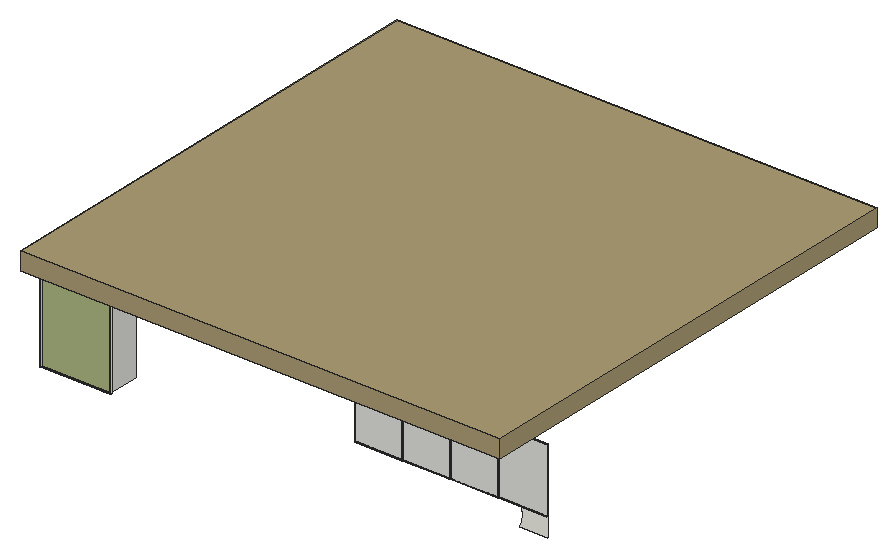
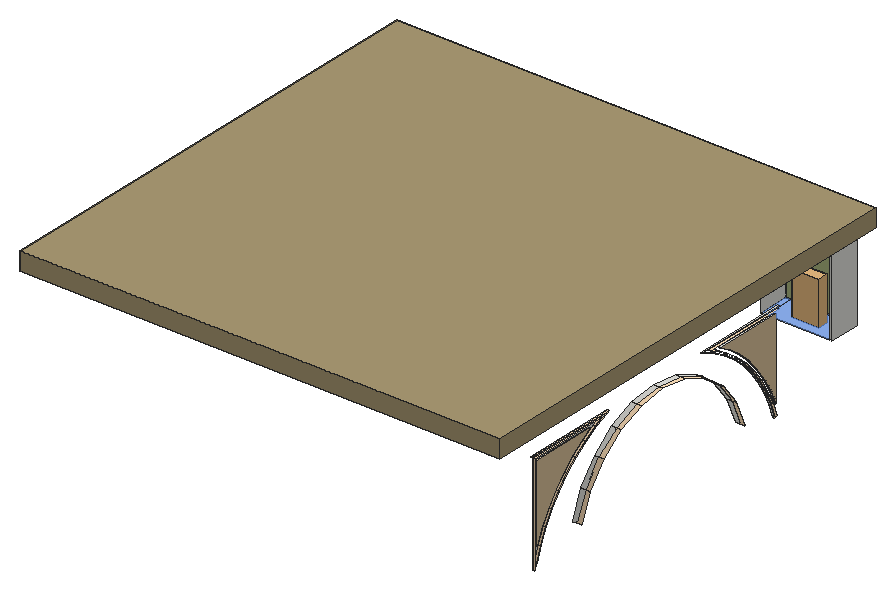
# SketchUp Ruby script. Lengths in inches.
U = 1.inch
M = Sketchup.active_model
def pt(a) = Geom::Point3d.new(a.map { |v| v * U })
def face(e, loops, mat)
  f = e.add_face(loops[0].map { |a| pt(a) })
  loops[1..].each { |l| e.add_face(l.map { |a| pt(a) }).erase! }
  f.material = f.back_material = mat if mat
  f
end
# faces: each face lists its corners as indices into pts; further lists are holes
def faces(e, pts, list, mat = nil) = list.each { |f| face(e, (f[0].is_a?(Array) ? f : [f]).map { |l| l.map { |i| pts[i] } }, mat) }
# xy, xz, yz: faces in a plane at the given z, y or x. An outline is a flat list of corners, or four numbers for a rectangle; further outlines are holes
def ring(l) = l.size == 4 ? [[l[0], l[1]], [l[2], l[1]], [l[2], l[3]], [l[0], l[3]]] : l.each_slice(2).to_a
def flat(e, list, mat, &to3) = list.each { |f| face(e, (f[0].is_a?(Array) ? f : [f]).map { |l| ring(l).map { |u, v| to3.(u, v) } }, mat) }
def xy(e, z, list, mat = nil) = flat(e, list, mat) { |x, y| [x, y, z] }
def xz(e, y, list, mat = nil) = flat(e, list, mat) { |x, z| [x, y, z] }
def yz(e, x, list, mat = nil) = flat(e, list, mat) { |y, z| [x, y, z] }
def lines(e, pts, list) = list.each { |a, b| e.add_line(pt(pts[a]), pt(pts[b])) }
# prism: a flat outline (further loops are holes) pulled along v
def prism(e, loops, v, mat = nil)
  f = face(e, loops, mat); d = Geom::Vector3d.new(v.map { |x| x * U })
  f.pushpull(f.normal.samedirection?(d) ? d.length : -d.length)
end
def box(e, o, s, mat = nil) = prism(e, [[o, [o[0] + s[0], o[1], o[2]], [o[0] + s[0], o[1] + s[1], o[2]], [o[0], o[1] + s[1], o[2]]]], [0, 0, s[2]], mat)
def at(x, y, z, deg = 0) = Geom::Transformation.translation(pt([x, y, z])) * Geom::Transformation.rotation(ORIGIN, Z_AXIS, deg.degrees)
def axes(o, x, y, z) = Geom::Transformation.new([*x, 0, *y, 0, *z, 0, *pt(o).to_a, 1])
def part(name) = M.definitions.add(name)
# library, detail: a bought-in or finely detailed component or shape, given as its bounding box
def library(name, o, s) = part(name).tap { |d| box(d.entities, o, s) }
def detail(e, o, s) = box(e.add_group.entities, o, s)
def put(e, d, t, mat = nil) = e.add_instance(d, t).tap { |i| i.material = mat if mat }
def group(e, t, mat = nil) = e.add_group.tap { |g| g.transformation = t; g.material = mat if mat }.entities
root = M.entities
M.materials.add("BACK Wall colour").color = [219, 194, 155]
M.materials.add("Emissive").color = [255, 225, 187]
M.materials.add("Emissive\#1").color = [255, 255, 255]
M.materials.add("[Color A01]").color = [173, 157, 118]
M.materials.add("[Translucent Glass Blue]").color = [100, 149, 237]
M.materials["[Translucent Glass Blue]"].alpha = 0.5
M.materials.add("celling colour").color = [232, 202, 161]
M.materials.add("cubod").color = [174, 185, 130]
M.materials.add("cubod wall").color = [240, 240, 232]
c1 = library("Group\#137",[0,0,0],[10.08,3.9375,16.2])
c2 = library("Ceiling Lamp 298 005",[-48.92,-48.77,-111.12],[97.53,97.41,111.46])
c3 = part("Component\#3")
detail(c3.entities,[-0.59,-0.59,-1.4375],[11.52,11.52,1.6875])
xy(root,93.69,[[688.79,27,706.63,27.75],[706.79,27,724.63,27.75]])
xy(root,94,[[589.4375,4,613.52,4.375],[613.52,4,615.39,4.375],[688.79,27,706.63,27.75],[706.79,27,724.63,27.75],[724.63,27,724.79,27.75]])
xy(root,94,[[589.4375,4.375,613.52,16],[613.52,4.375,615.39,16]],"[Translucent Glass Blue]")
xy(root,94.39,[[589.4375,4,615.39,4.375]])
xy(root,94.39,[[589.4375,4.375,615.39,16]],"[Translucent Glass Blue]")
xy(root,115.1875,[[588.45,43.01,588.79,68.75],[588.42,130.16,588.79,155.1875]])
xy(root,115.1875,[[588.1,43.01,588.45,68.75],[588.1,130.16,588.42,155.1875]],"Emissive")
xy(root,116.375,[[588.1,41.82,588.79,73.63],[588.1,125.18,588.79,156.375]],"Emissive")
xy(root,117.17,[[588.45,41.03,588.79,77.31],[588.45,121.42,588.79,157.17]])
xy(root,117.17,[[588.1,41.03,588.45,77.31],[588.1,121.42,588.45,157.17]],"Emissive")
xy(root,118,[[688.79,27,706.63,27.75],[706.79,27,724.63,27.75],[724.79,27,742.63,27.75],[742.79,27,760.79,27.75]])
xy(root,124,[[588.79,4,589.4375,16],[589.4375,4,615.39,4.375],[615.39,4,616.04,4.375],[615.39,4.375,616.04,16]])
xy(root,124,[[589.4375,4.375,615.39,16]],"[Translucent Glass Blue]")
xy(root,124.2,[[588.79,4,589.4375,4.375],[589.4375,4,616.04,4.375]])
xy(root,124.57,[[589.4375,4,616.04,16]],"[Translucent Glass Blue]")
xy(root,126.48,[[584.79,4,588.79,176.875]])
xz(root,4,[[589.4375,94,615.39,94.39],[615.39,94.39,616.04,124],[588.79,124,589.4375,124.2],[589.4375,124,616.04,124.2],[589.4375,124.2,616.04,124.57]])
xz(root,4.375,[[589.4375,94.39,615.39,124]],"cubod")
xz(root,16,[[589.4375,124,616.04,124.57]],"[Translucent Glass Blue]")
xz(root,27,[[688.79,93.69,706.79,94],[706.79,93.69,724.79,94],[724.79,93.69,742.63,94],[742.63,93.69,742.79,94],[742.79,93.69,760.79,94],
  [688.79,94,706.63,118],[706.63,94,706.79,118],[706.79,94,724.63,118],[724.63,94,724.79,118],[724.79,94,742.63,118],
  [742.63,94,742.79,118],[742.79,94,760.79,118]])
xz(root,27.75,[[688.79,94,688.79,100.05,688.86,100.89,689.08,101.7,689.44,102.46,689.93,103.15,690.53,103.74,691.23,104.22,691.99,104.56,692.81,104.77,693.65,104.83,694.49,104.75,695.3,104.51,696.05,104.14,696.4,106.79,697.42,109.25,699.04,111.37,701.16,112.99,703.625,114.01,706.27,114.36,706.63,114.32,706.63,94],[706.79,94,706.79,114.29,708.92,114.01,711.38,112.99,713.5,111.37,715.12,109.25,716.14,106.79,716.49,104.14,717.99,106.42,720.03,108.23,722.47,109.44,724.63,109.89,724.63,94]],"cubod")
xz(root,27.75,[[750.1,86.35,750.97,88.41,751.28,90.64,750.99,92.86,750.15,94.9375,748.79,96.73,747.02,98.1,744.95,98.97,742.79,99.26,742.79,118,760.79,118,760.79,86.35],[735.26,95.01,736.125,97.6,736.29,100.32,735.74,102.99,734.52,105.42,732.71,107.46,730.44,108.97,727.86,109.83,725.14,109.99,724.79,109.92,724.79,118,742.63,118,742.63,99.26,740.5,98.99,738.42,98.14,736.64,96.79],[688.79,100.05,688.79,118,706.63,118,706.63,114.32,706.27,114.36,703.625,114.01,701.16,112.99,699.04,111.37,697.42,109.25,696.4,106.79,696.05,104.14,695.3,104.51,694.49,104.75,693.65,104.83,692.81,104.77,691.99,104.56,691.23,104.22,690.53,103.74,689.93,103.15,689.44,102.46,689.08,101.7,688.86,100.89],[716.49,104.14,716.14,106.79,715.12,109.25,713.5,111.37,711.38,112.99,708.92,114.01,706.79,114.29,706.79,118,724.63,118,724.63,109.89,722.47,109.44,720.03,108.23,717.99,106.42]],"cubod wall")
xz(root,43.01,[[588.45,85.13,588.79,115.1875]])
xz(root,43.01,[[588.1,85.13,588.45,115.1875]],"Emissive")
xz(root,155.1875,[[588.42,86.57,588.79,115.1875]])
xz(root,155.1875,[[588.1,86.57,588.42,115.1875]],"Emissive")
xz(root,156.375,[[588.1,78.67,588.79,116.375]],"Emissive")
yz(root,588.1,[[43.01,85.13,43.52,86.57,45.99,91.8,48.96,96.77,52.41,101.42,56.29,105.71,60.57,109.6,65.21,113.06,68.75,115.1875,43.01,115.1875],[155.1875,86.57,155.1875,115.1875,130.16,115.1875,133.5625,113.1875,138.23,109.76,142.53,105.87,146.41,101.57,149.84,96.89,152.77,91.89,155.17,86.62]],"BACK Wall colour")
yz(root,588.79,[[[156.375,78.67,156.375,116.375,125.18,116.375,128.02,115.07,132.91,112.2,137.48,108.84,141.69,105.03,145.49,100.82,148.84,96.24,151.71,91.34,154.07,86.18,155.89,80.81],[155.1875,86.57,155.17,86.62,152.77,91.89,149.84,96.89,146.41,101.57,142.53,105.87,138.23,109.76,133.5625,113.1875,130.16,115.1875,155.1875,115.1875]],[4,94,16,124],[4,124,16,124.2],[4,124.2,16,126.48]])
yz(root,589.4375,[[4,94.39,4.375,124],[4.375,94.39,16,124],[4.375,124,4.375,124.2,4,124.2,4,124.57,16,124.57,16,124]])
yz(root,615.39,[[4,94.39,4.375,124],[4.375,94.39,16,124]])
yz(root,616.04,[[4,124,16,124.2],[4,124.2,16,124.57]],"[Translucent Glass Blue]")
yz(root,688.79,[[27,94,27.75,118]])
yz(root,706.63,[[27,94,27.75,118]])
yz(root,706.79,[[27,94,27.75,118]])
yz(root,724.63,[[27,94,27.75,118]])
yz(root,724.79,[[27,93.69,27.75,94],[27,94,27.75,118]])
yz(root,742.63,[[27,93.69,27.75,94],[27,94,27.75,118]])
yz(root,742.79,[[27,93.69,27.75,94],[27,94,27.75,118]])
p = [[588.79,156.375,78.67],[588.79,155.89,80.81],[588.1,155.89,80.81],[588.1,156.375,78.67],[588.1,43.48,80.54],[588.45,43.48,80.54],
  [588.45,45.36,85.81],[588.1,45.36,85.81],[588.79,45.36,85.81],[588.79,43.48,80.54],[588.1,153.33,85.89],[588.45,153.33,85.89],
  [588.45,155.12,80.59],[588.1,155.12,80.59],[588.79,155.12,80.59],[588.79,153.33,85.89],[588.79,44.62,86.11],[588.79,42.71,80.77],
  [588.1,42.71,80.77],[588.1,44.62,86.11],[588.79,154.07,86.18],[588.1,154.07,86.18],[588.1,43.01,85.13],[588.45,43.01,85.13],
  [588.45,43.52,86.57],[588.1,43.52,86.57],[588.79,43.52,86.57],[588.79,43.01,85.13],[588.45,47.74,90.87],[588.1,47.74,90.87],
  [588.79,47.74,90.87],[588.1,151,90.98],[588.45,151,90.98],[588.79,151,90.98],[588.79,47.04,91.24],[588.1,47.04,91.24],
  [588.79,151.71,91.34],[588.1,151.71,91.34],[588.45,45.99,91.8],[588.1,45.99,91.8],[588.79,45.99,91.8],[588.1,152.77,91.89],
  [588.42,152.77,91.89],[588.42,155.17,86.62],[588.1,155.17,86.62],[588.79,155.17,86.62],[588.79,152.77,91.89],[588.42,155.1875,86.57],
  [588.1,155.1875,86.57],[588.79,155.1875,86.57],[585.35,65.14,96.27],[587.07,65.14,96.27],[587.07,61.19,86.73],[585.35,61.19,86.73],
  [588.79,61.19,86.73],[588.79,65.14,96.27],[585.35,137.54,86.73],[587.07,137.54,86.73],[587.07,133.59,96.27],[585.35,133.59,96.27],
  [588.79,133.59,96.27],[588.79,137.54,86.73],[588.45,50.61,95.67],[588.1,50.61,95.67],[588.79,50.61,95.67],[588.1,148.18,95.8],
  [588.45,148.18,95.8],[588.79,148.18,95.8],[588.79,49.95,96.11],[588.1,49.95,96.11],[588.79,148.84,96.24],[588.1,148.84,96.24],
  [588.45,48.96,96.77],[588.1,48.96,96.77],[588.79,48.96,96.77],[588.1,149.84,96.89],[588.42,149.84,96.89],[588.79,149.84,96.89],
  [588.45,53.94,100.16],[588.1,53.94,100.16],[588.79,53.94,100.16],[588.1,144.87,100.31],[588.45,144.87,100.31],[588.79,144.87,100.31],
  [588.79,53.33,100.67],[588.1,53.33,100.67],[588.79,145.49,100.82],[588.1,145.49,100.82],[585.35,71.42,104.45],[587.07,71.42,104.45],
  [588.79,71.42,104.45],[587.07,127.31,104.45],[585.35,127.31,104.45],[588.79,127.31,104.45],[588.45,52.41,101.42],[588.1,52.41,101.42],
  [588.79,52.41,101.42],[588.1,146.41,101.57],[588.42,146.41,101.57],[588.79,146.41,101.57],[588.45,57.69,104.3125],[588.1,57.69,104.3125],
  [588.79,57.69,104.3125],[588.1,141.13,104.47],[588.45,141.13,104.47],[588.79,141.13,104.47],[588.79,57.13,104.875],[588.1,57.13,104.875],
  [588.79,141.69,105.03],[588.1,141.69,105.03],[588.45,56.29,105.71],[588.1,56.29,105.71],[588.79,56.29,105.71],[588.1,142.53,105.87],
  [588.42,142.53,105.87],[588.79,142.53,105.87],[588.45,61.83,108.07],[588.1,61.83,108.07],[588.79,61.83,108.07],[585.35,79.6,110.73],
  [587.07,79.6,110.73],[588.79,79.6,110.73],[587.07,119.125,110.73],[585.35,119.125,110.73],[588.79,119.125,110.73],[588.1,136.98,108.22],
  [588.45,136.98,108.22],[588.79,136.98,108.22],[588.79,61.32,108.6875],[588.1,61.32,108.6875],[588.79,137.48,108.84],[588.1,137.48,108.84],
  [588.45,60.57,109.6],[588.1,60.57,109.6],[588.79,60.57,109.6],[588.1,138.23,109.76],[588.42,138.23,109.76],[588.79,138.23,109.76],
  [588.45,66.32,111.41],[588.1,66.32,111.41],[588.79,66.32,111.41],[588.1,132.47,111.53],[588.45,132.47,111.53],[588.79,132.47,111.53],
  [588.79,65.875,112.07],[588.1,65.875,112.07],[588.79,132.91,112.2],[588.1,132.91,112.2],[588.45,65.21,113.06],[588.1,65.21,113.06],
  [588.79,65.21,113.06],[588.1,133.5625,113.1875],[588.42,133.5625,113.1875],[588.79,133.5625,113.1875],[585.35,89.14,114.68],[587.07,89.14,114.68],
  [588.79,89.14,114.68],[587.07,109.59,114.68],[585.35,109.59,114.68],[588.79,109.59,114.68],[588.45,71.11,114.29],[588.1,71.11,114.29],
  [588.79,71.11,114.29],[588.1,127.65,114.37],[588.45,127.65,114.37],[588.79,127.65,114.37],[588.79,70.73,115],[588.1,70.73,115],
  [588.79,128.02,115.07],[588.1,128.02,115.07],[588.45,68.75,115.1875],[588.1,68.75,115.1875],[588.79,68.75,115.1875],[588.1,130.16,115.1875],
  [588.42,130.16,115.1875],[588.79,130.16,115.1875],[588.45,76.16,116.7],[588.1,76.16,116.7],[588.79,76.16,116.7],[588.1,122.57,116.7],
  [588.45,122.57,116.7],[588.79,122.57,116.7],[585.35,99.36,116.03],[587.07,99.36,116.03],[588.79,99.36,116.03],[588.79,73.63,116.375],
  [588.1,73.63,116.375],[588.79,125.18,116.375],[588.1,125.18,116.375],[588.45,77.31,117.17],[588.1,77.31,117.17],[588.79,77.31,117.17],
  [588.1,121.42,117.17],[588.45,121.42,117.17],[588.79,121.42,117.17],[724.79,27.75,109.92],[724.63,27.75,109.89],[706.79,27.75,114.29],
  [706.63,27.75,114.32],[742.73,27.75,99.27],[742.63,27.75,99.26],[742.79,27.75,99.26],[742.63,27.75,118],[742.79,27.75,118]]
faces(root,p,[[0,1,2,3],[4,5,6,7],[10,11,12,13],[16,17,18,19],[1,20,21,2],[22,23,24,25],[7,6,28,29],[31,32,11,10],
  [34,16,19,35],[20,36,37,21],[25,24,38,39],[41,42,43,44],[44,43,47,48],[50,51,52,53],[56,57,58,59],[29,28,62,63],
  [65,66,32,31],[68,34,35,69],[36,70,71,37],[39,38,72,73],[75,76,42,41],[63,62,78,79],[81,82,66,65],[84,68,69,85],
  [70,86,87,71],[88,89,51,50],[59,58,91,92],[73,72,94,95],[97,98,76,75],[79,78,100,101],[103,104,82,81],[106,84,85,107],
  [86,108,109,87],[95,94,110,111],[113,114,98,97],[101,100,116,117],[119,120,89,88],[92,91,122,123],[125,126,104,103],[128,106,107,129],
  [108,130,131,109],[111,110,132,133],[135,136,114,113],[117,116,138,139],[141,142,126,125],[144,128,129,145],[130,146,147,131],[133,132,148,149],
  [151,152,136,135],[154,155,120,119],[123,122,157,158],[139,138,160,161],[163,164,142,141],[166,144,145,167],[146,168,169,147],[149,148,170,171],
  [173,174,152,151],[161,160,176,177],[179,180,164,163],[182,183,155,154],[158,157,183,182],[185,166,167,186],[168,187,188,169],[177,176,189,190],
  [192,193,180,179]],"Emissive")
faces(root,p,[[8,6,5,9],[14,12,11,15],[26,24,23,27],[30,28,6,8],[15,11,32,33],[40,38,24,26],[45,43,42,46],[49,47,43,45],
  [54,52,51,55],[60,58,57,61],[64,62,28,30],[33,32,66,67],[74,72,38,40],[46,42,76,77],[80,78,62,64],[67,66,82,83],
  [55,51,89,90],[93,91,58,60],[96,94,72,74],[77,76,98,99],[102,100,78,80],[83,82,104,105],[112,110,94,96],[99,98,114,115],
  [118,116,100,102],[90,89,120,121],[124,122,91,93],[105,104,126,127],[134,132,110,112],[115,114,136,137],[140,138,116,118],[127,126,142,143],
  [150,148,132,134],[137,136,152,153],[121,120,155,156],[159,157,122,124],[162,160,138,140],[143,142,164,165],[172,170,148,150],[153,152,174,175],
  [178,176,160,162],[165,164,180,181],[156,155,183,184],[184,183,157,159],[191,189,176,178],[181,180,193,194]])
lines(root,p,[[195,196],[197,198],[199,200],[201,199],[202,203]])
put(root,c1,at(606.5,12.53,94.39,180))
put(root,c2,axes([663.66,98.67,131.84],[0.279,0,0],[0,0.279,0],[0,0,0.279]))
g1 = group(root,at(588.79,23.29,135.52),"[Color A01]")
xy(g1,-9.04,[[[-4,-23.29,176,153.59],[24.9375,23.99,24.49,24.02,24.04,24.1,23.62,24.25,23.21,24.45,22.84,24.7,22.5,25,22.2,25.34,21.95,25.71,21.75,26.12,21.6,26.55,21.51,26.99,21.48,27.44,21.48,127.94,21.51,128.39,21.6,128.84,21.75,129.26,21.95,129.67,22.2,130.04,22.5,130.38,22.84,130.68,23.21,130.93,23.62,131.13,24.04,131.28,24.49,131.37,24.9375,131.4,136.36,131.4,136.81,131.37,137.25,131.28,137.68,131.13,138.09,130.93,138.46,130.68,138.8,130.38,139.1,130.04,139.35,129.67,139.55,129.26,139.7,128.84,139.78,128.39,139.8125,127.94,139.8125,27.44,139.78,26.99,139.7,26.55,139.55,26.12,139.35,25.71,139.1,25.34,138.8,25,138.46,24.7,138.09,24.45,137.68,24.25,137.25,24.1,136.81,24.02,136.36,23.99]]],"celling colour")
xy(g1,-3.58,[[16.72,19.28,144.52,133.6]],"celling colour")
xy(g1,-2.25,[[-4,-23.29,176,153.59]],"[Color A01]")
xz(g1,-23.29,[[-4,-9.04,176,-2.25]])
xz(g1,19.28,[[16.72,-6.3125,144.52,-3.58]],"Emissive\#1")
xz(g1,23.99,[[24.9375,-9.04,136.36,-6.43]],"[Color A01]")
xz(g1,131.4,[[24.9375,-9.04,136.36,-6.43]],"[Color A01]")
xz(g1,133.6,[[16.72,-6.3125,144.52,-3.58]],"Emissive\#1")
xz(g1,153.59,[[-4,-9.04,176,-2.25]],"[Color A01]")
yz(g1,-4,[[-23.29,-9.04,153.59,-2.25]])
yz(g1,16.72,[[19.28,-6.3125,133.6,-3.58]],"Emissive\#1")
yz(g1,21.48,[[27.44,-9.04,127.94,-6.43]])
yz(g1,139.8125,[[27.44,-9.04,127.94,-6.43]],"[Color A01]")
yz(g1,144.52,[[19.28,-6.3125,133.6,-3.58]],"Emissive\#1")
yz(g1,176,[[-23.29,-9.04,153.59,-2.25]])
p = [[24.04,24.1,-9.04],[24.49,24.02,-9.04],[24.49,24.02,-6.43],[24.04,24.1,-6.43],[24.9375,23.99,-9.04],[24.9375,23.99,-6.43],
  [136.36,23.99,-9.04],[136.81,24.02,-9.04],[136.81,24.02,-6.43],[136.36,23.99,-6.43],[137.25,24.1,-9.04],[137.25,24.1,-6.43],
  [23.62,24.25,-9.04],[23.62,24.25,-6.43],[137.68,24.25,-9.04],[137.68,24.25,-6.43],[23.21,24.45,-9.04],[23.21,24.45,-6.43],
  [138.09,24.45,-9.04],[138.09,24.45,-6.43],[22.84,24.7,-9.04],[22.84,24.7,-6.43],[138.46,24.7,-9.04],[138.46,24.7,-6.43],
  [22.5,25,-9.04],[22.5,25,-6.43],[138.8,25,-9.04],[138.8,25,-6.43],[22.2,25.34,-9.04],[22.2,25.34,-6.43],
  [139.1,25.34,-9.04],[139.1,25.34,-6.43],[21.95,25.71,-9.04],[21.95,25.71,-6.43],[139.35,25.71,-9.04],[139.35,25.71,-6.43],
  [21.75,26.12,-9.04],[21.75,26.12,-6.43],[139.55,26.12,-9.04],[139.55,26.12,-6.43],[21.6,26.55,-9.04],[21.6,26.55,-6.43],
  [139.7,26.55,-9.04],[139.7,26.55,-6.43],[21.51,26.99,-9.04],[21.51,26.99,-6.43],[139.78,26.99,-9.04],[139.78,26.99,-6.43],
  [21.48,27.44,-9.04],[21.48,27.44,-6.43],[139.8125,27.44,-9.04],[139.8125,27.44,-6.43],[21.51,128.39,-9.04],[21.48,127.94,-9.04],
  [21.48,127.94,-6.43],[21.51,128.39,-6.43],[139.8125,127.94,-9.04],[139.78,128.39,-9.04],[139.78,128.39,-6.43],[139.8125,127.94,-6.43],
  [21.6,128.84,-9.04],[21.6,128.84,-6.43],[139.7,128.84,-9.04],[139.7,128.84,-6.43],[21.75,129.26,-9.04],[21.75,129.26,-6.43],
  [139.55,129.26,-9.04],[139.55,129.26,-6.43],[21.95,129.67,-9.04],[21.95,129.67,-6.43],[139.35,129.67,-9.04],[139.35,129.67,-6.43],
  [22.2,130.04,-9.04],[22.2,130.04,-6.43],[139.1,130.04,-9.04],[139.1,130.04,-6.43],[22.5,130.38,-9.04],[22.5,130.38,-6.43],
  [138.8,130.38,-9.04],[138.8,130.38,-6.43],[22.84,130.68,-9.04],[22.84,130.68,-6.43],[138.46,130.68,-9.04],[138.46,130.68,-6.43],
  [23.21,130.93,-9.04],[23.21,130.93,-6.43],[138.09,130.93,-9.04],[138.09,130.93,-6.43],[23.62,131.13,-9.04],[23.62,131.13,-6.43],
  [137.68,131.13,-9.04],[137.68,131.13,-6.43],[24.04,131.28,-9.04],[24.04,131.28,-6.43],[137.25,131.28,-9.04],[137.25,131.28,-6.43],
  [24.49,131.37,-9.04],[24.49,131.37,-6.43],[136.81,131.37,-9.04],[136.81,131.37,-6.43],[24.9375,131.4,-9.04],[24.9375,131.4,-6.43],
  [136.36,131.4,-9.04],[136.36,131.4,-6.43],[141.96,26.85,-6.3125],[141.96,19.28,-6.3125]]
faces(g1,p,[[0,1,2,3],[1,4,5,2],[12,0,3,13],[16,12,13,17],[20,16,17,21],[24,20,21,25],[28,24,25,29],[32,28,29,33],
  [36,32,33,37],[40,36,37,41],[44,40,41,45],[48,44,45,49],[52,53,54,55],[60,52,55,61],[64,60,61,65],[68,64,65,69],
  [72,68,69,73],[76,72,73,77],[80,76,77,81],[84,80,81,85],[88,84,85,89],[92,88,89,93],[96,92,93,97],[100,96,97,101]])
faces(g1,p,[[6,7,8,9],[7,10,11,8],[10,14,15,11],[14,18,19,15],[18,22,23,19],[22,26,27,23],[26,30,31,27],[30,34,35,31],
  [34,38,39,35],[38,42,43,39],[42,46,47,43],[46,50,51,47],[56,57,58,59],[57,62,63,58],[62,66,67,63],[66,70,71,67],
  [70,74,75,71],[74,78,79,75],[78,82,83,79],[82,86,87,83],[86,90,91,87],[90,94,95,91],[94,98,99,95],[98,102,103,99]],"[Color A01]")
lines(g1,p,[[104,105]])
put(g1,c3,axes([6.95,7.53,-9.04],[0.88861,0,0],[0,0.88861,0],[0,0,-0.88861]))
put(g1,c3,axes([147.4,7.84,-9.04],[0.8281,0,0],[0,0.8281,0],[0,0,-0.8281]))
put(g1,c3,axes([7.24,137.48,-9.04],[0.81757,0,0],[0,0.81757,0],[0,0,-0.81757]))
put(g1,c3,axes([146.51,134.45,-9.04],[0.8099,0,0],[0,0.8099,0],[0,0,-0.8099]))
